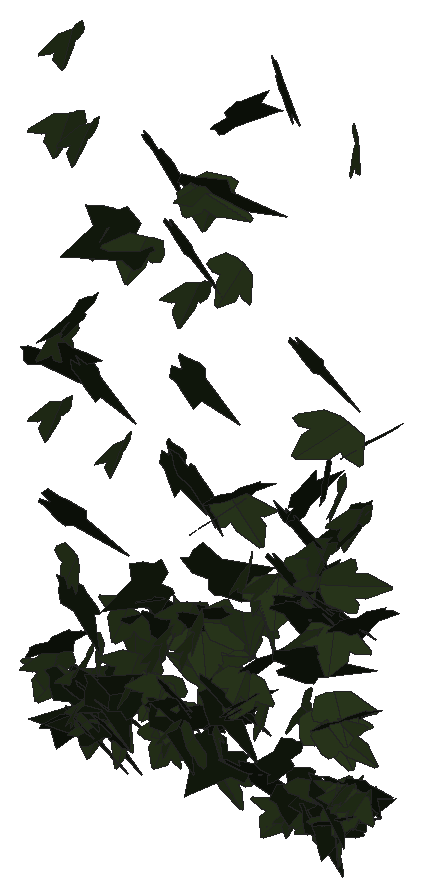
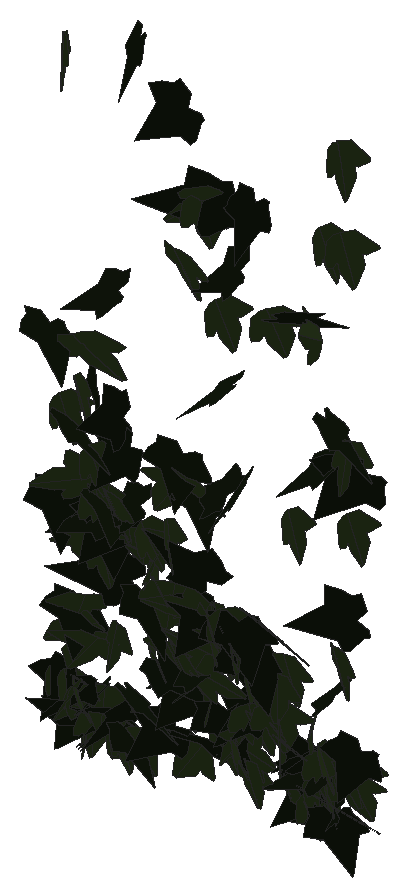
# SketchUp Ruby script. Lengths in inches.
U = 1.inch
M = Sketchup.active_model
def pt(a) = Geom::Point3d.new(a.map { |v| v * U })
def face(e, loops, mat)
  f = e.add_face(loops[0].map { |a| pt(a) })
  loops[1..].each { |l| e.add_face(l.map { |a| pt(a) }).erase! }
  f.material = f.back_material = mat if mat
  f
end
# faces: each face lists its corners as indices into pts; further lists are holes
def faces(e, pts, list, mat = nil) = list.each { |f| face(e, (f[0].is_a?(Array) ? f : [f]).map { |l| l.map { |i| pts[i] } }, mat) }
# xy, xz, yz: faces in a plane at the given z, y or x. An outline is a flat list of corners, or four numbers for a rectangle; further outlines are holes
def ring(l) = l.size == 4 ? [[l[0], l[1]], [l[2], l[1]], [l[2], l[3]], [l[0], l[3]]] : l.each_slice(2).to_a
def flat(e, list, mat, &to3) = list.each { |f| face(e, (f[0].is_a?(Array) ? f : [f]).map { |l| ring(l).map { |u, v| to3.(u, v) } }, mat) }
def xy(e, z, list, mat = nil) = flat(e, list, mat) { |x, y| [x, y, z] }
def xz(e, y, list, mat = nil) = flat(e, list, mat) { |x, z| [x, y, z] }
def yz(e, x, list, mat = nil) = flat(e, list, mat) { |y, z| [x, y, z] }
def lines(e, pts, list) = list.each { |a, b| e.add_line(pt(pts[a]), pt(pts[b])) }
# prism: a flat outline (further loops are holes) pulled along v
def prism(e, loops, v, mat = nil)
  f = face(e, loops, mat); d = Geom::Vector3d.new(v.map { |x| x * U })
  f.pushpull(f.normal.samedirection?(d) ? d.length : -d.length)
end
def box(e, o, s, mat = nil) = prism(e, [[o, [o[0] + s[0], o[1], o[2]], [o[0] + s[0], o[1] + s[1], o[2]], [o[0], o[1] + s[1], o[2]]]], [0, 0, s[2]], mat)
def at(x, y, z, deg = 0) = Geom::Transformation.translation(pt([x, y, z])) * Geom::Transformation.rotation(ORIGIN, Z_AXIS, deg.degrees)
def axes(o, x, y, z) = Geom::Transformation.new([*x, 0, *y, 0, *z, 0, *pt(o).to_a, 1])
def part(name) = M.definitions.add(name)
# library, detail: a bought-in or finely detailed component or shape, given as its bounding box
def library(name, o, s) = part(name).tap { |d| box(d.entities, o, s) }
def detail(e, o, s) = box(e.add_group.entities, o, s)
def put(e, d, t, mat = nil) = e.add_instance(d, t).tap { |i| i.material = mat if mat }
def group(e, t, mat = nil) = e.add_group.tap { |g| g.transformation = t; g.material = mat if mat }.entities
root = M.entities
M.materials.add("1026 AP 7946 SUNNY SIDE UP").color = [254, 231, 186]
M.materials.add("efeu1").color = [18, 25, 13]
M.materials.add("efeu2").color = [43, 57, 29]
c1 = part("ivyleaf_10")
p = [[0,0.5,-0.03],[-0.0625,2.02,-0.43],[-0.19,2.01,-0.46],[-0.54,1.05,-0.29],[-0.52,0.625,-0.18],[-0.83,0.76,-0.28],
  [-1.16,0.64,-0.33],[-1.15,0.33,-0.24],[-0.77,-0.39,0.02],[-0.3,-0.51,0.16],[0.04,-0.48,0.23],[-0.02,2.01,-0.4375],
  [-0.06,2.01,-0.43],[0.04,-0.49,0.23],[0.67,-0.49,0.14],[1.38,0.36,-0.2],[1.375,0.51,-0.24],[0.81,0.65,-0.19],
  [0.62,0.59,-0.15],[0.6,1.09,-0.28],[0.5,1.23,-0.31]]
faces(c1.entities,p,[[0,1,2,3,4,5,6,7,8,9,10],[11,12,0,13,14,15,16,17,18,19,20]],"efeu2")
c2 = part("ivyleaf_9")
p = [[1.54,2.16,1.25],[1.36,2.04,1.19],[-0.21,0.99,0.68],[-0.71,1.11,0.82],[-0.85,0.86,0.67],[-0.8,0.17,0.21],
  [-0.9,-0.01,0.1],[-0.67,-0.16,-0.02],[-0.08,-0.08,-0.05],[-0.03,-0.6,-0.4],[0.65,-0.88,-0.66],[0.83,-0.6,-0.49],
  [1.29,-0.42,-0.43],[1.8125,-0.07,-0.26],[1.21,0.44,0.15]]
faces(c2.entities,p,[[0,1,2,3,4,5,6,7,8,9,10,11,12,13,14]],"efeu1")
put(root,c1,axes([113.07,212.89,268.62],[-0.34334,-0.07653,0.12729],[-0.15139,-0.09188,-0.23364],[0.17197,-0.23369,0.04845]),"1026 AP 7946 SUNNY SIDE UP")
put(root,c2,axes([112.96,212.81,269.11],[0.15845,0.23705,0.05643],[0.06227,0.04104,-0.26432],[-0.37697,0.10642,-0.01995]),"1026 AP 7946 SUNNY SIDE UP")
put(root,c1,axes([113.02,212.83,268.85],[-0.17621,-0.24452,0.01132],[0.00626,-0.01543,-0.27699],[0.38492,-0.11169,0.00969]),"1026 AP 7946 SUNNY SIDE UP")
put(root,c1,axes([113.06,212.85,272.75],[-0.06958,-0.28014,0.02649],[-0.00163,-0.02748,-0.29232],[0.44258,-0.04414,0.00309]),"1026 AP 7946 SUNNY SIDE UP")
put(root,c2,axes([112.92,212.8125,273.57],[0.40205,0.1369,0.01777],[0.04671,-0.0208,-0.29705],[-0.21173,0.25537,-0.03179]),"1026 AP 7946 SUNNY SIDE UP")
put(root,c1,axes([113.18,212.87,277.2],[-0.16313,-0.28328,0.03071],[-0.00181,-0.03302,-0.3108],[0.44816,-0.10325,0.00992]),"1026 AP 7946 SUNNY SIDE UP")
put(root,c1,axes([113.14,212.82,273.87],[-0.08095,-0.26244,-0.12112],[0.06477,0.10995,-0.27427],[0.44654,-0.06352,0.01783]),"1026 AP 7946 SUNNY SIDE UP")
put(root,c2,axes([113.29,212.93,268.01],[0.07076,0.22691,-0.1179],[-0.02317,-0.11501,-0.23888],[-0.39986,0.04682,-0.00702]),"1026 AP 7946 SUNNY SIDE UP")
put(root,c2,axes([113.42,212.92,274.29],[-0.26406,0.22273,-0.07554],[0.04809,-0.07017,-0.28723],[-0.36619,-0.16983,0.01675]),"1026 AP 7946 SUNNY SIDE UP")
put(root,c1,axes([113.29,212.8,278.58],[-0.06665,-0.30699,-0.03908],[0.01318,0.03537,-0.31903],[0.48587,-0.04307,0.00329]),"1026 AP 7946 SUNNY SIDE UP")
put(root,c1,axes([113.35,212.78,270.5],[0.28252,-0.18935,-0.09053],[-0.04399,0.09166,-0.2651],[0.32456,0.17724,0.04287]),"1026 AP 7946 SUNNY SIDE UP")
put(root,c2,axes([113.02,212.85,271.23],[0.40541,-0.07099,0.12199],[0.16962,-0.05435,-0.27491],[0.13637,0.27864,-0.02074]),"1026 AP 7946 SUNNY SIDE UP")
put(root,c2,axes([113.21,212.91,268.62],[0.1171,-0.24383,-0.06473],[0.0273,0.06892,-0.25965],[0.39444,0.06762,0.03719]),"1026 AP 7946 SUNNY SIDE UP")
put(root,c1,axes([113.47,212.97,268.98],[0.08636,-0.25577,-0.01492],[-0.00783,0.01225,-0.26941],[0.40261,0.0551,-0.00204]),"1026 AP 7946 SUNNY SIDE UP")
put(root,c1,axes([113.47,212.83,268.35],[0.09709,-0.25754,-0.02951],[-0.00239,0.02758,-0.27262],[0.4072,0.06157,0.00543]),"1026 AP 7946 SUNNY SIDE UP")
put(root,c2,axes([113.79,212.85,268.17],[-0.33733,0.12121,0.10169],[-0.18391,-0.01491,-0.24479],[-0.16205,-0.23539,0.06612]),"1026 AP 7946 SUNNY SIDE UP")
put(root,c1,axes([113.52,212.875,277.17],[-0.02665,-0.30085,0.02682],[0.00126,-0.02783,-0.31058],[0.47506,-0.01681,0.00233]),"1026 AP 7946 SUNNY SIDE UP")
put(root,c2,axes([113.3125,212.93,269.96],[0.12745,-0.25297,0.03802],[0.00317,-0.03958,-0.2737],[0.40231,0.08045,-0.00989]),"1026 AP 7946 SUNNY SIDE UP")
put(root,c1,axes([113.58,212.88,268.8],[-0.18225,-0.23438,0.02402],[-0.00157,-0.02697,-0.26929],[0.37058,-0.11538,0.01067]),"1026 AP 7946 SUNNY SIDE UP")
put(root,c1,axes([113.67,212.87,268.39],[-0.07062,-0.25386,0.05692],[-0.01363,-0.05604,-0.26591],[0.40878,-0.04573,0.00097]),"1026 AP 7946 SUNNY SIDE UP")
put(root,c2,axes([113.39,212.87,268.07],[0.29729,-0.17873,0.03698],[0.05446,-0.01704,-0.26788],[0.28175,0.19188,0.01276]),"1026 AP 7946 SUNNY SIDE UP")
put(root,c1,axes([113.75,212.88,268.07],[-0.12803,-0.24599,0.03851],[-0.00362,-0.04005,-0.26696],[0.39156,-0.0808,0.01012]),"1026 AP 7946 SUNNY SIDE UP")
put(root,c1,axes([113.74,212.83,275.46],[0.17141,-0.14666,0.23722],[-0.14205,0.21554,0.18608],[-0.40627,-0.13724,0.03503]),"1026 AP 7946 SUNNY SIDE UP")
put(root,c2,axes([113.52,212.82,273.53],[0.33045,-0.17427,-0.09502],[-0.06233,0.09327,-0.27701],[0.30296,0.20927,0.04665]),"1026 AP 7946 SUNNY SIDE UP")
put(root,c2,axes([113.58,212.87,268.61],[0.35341,-0.14067,-0.01334],[0.04221,0.06499,-0.26329],[0.21797,0.2155,0.07261]),"1026 AP 7946 SUNNY SIDE UP")
put(root,c1,axes([113.7,212.96,269.18],[-0.02021,-0.03412,0.2681],[0.24776,-0.20962,-0.02151],[0.33044,0.15509,0.03253]),"1026 AP 7946 SUNNY SIDE UP")
put(root,c2,axes([114.2,213.01,275.72],[-0.35864,-0.09947,0.15449],[-0.17234,-0.11634,-0.25097],[0.22534,-0.24728,0.05393]),"1026 AP 7946 SUNNY SIDE UP")
put(root,c2,axes([113.78,212.79,268.54],[-0.13821,-0.02625,0.25803],[0.37194,-0.10009,0.07408],[0.13658,0.246,0.05937]),"1026 AP 7946 SUNNY SIDE UP")
put(root,c2,axes([113.84,212.8,268.17],[0.37975,-0.08446,-0.05098],[-0.08165,-0.00036,-0.26299],[0.13004,0.24643,-0.01625]),"1026 AP 7946 SUNNY SIDE UP")
put(root,c1,axes([114.07,212.92,272.48],[-0.01386,-0.27988,-0.02],[-0.00139,0.01786,-0.28837],[0.44097,-0.00874,-0.00154]),"1026 AP 7946 SUNNY SIDE UP")
put(root,c2,axes([113.9375,212.88,268.74],[0.0277,-0.25783,-0.06307],[-0.00826,0.05953,-0.26588],[0.41607,0.01835,-0.00108]),"1026 AP 7946 SUNNY SIDE UP")
put(root,c2,axes([114.35,212.86,268.85],[-0.39494,0.09218,0.00444],[-0.02265,-0.02831,-0.27387],[-0.14329,-0.2496,0.03103]),"1026 AP 7946 SUNNY SIDE UP")
put(root,c1,axes([114.32,212.79,270.04],[-0.39229,0.06098,0.10056],[-0.16882,-0.04153,-0.25711],[-0.06393,-0.26453,0.06188]),"1026 AP 7946 SUNNY SIDE UP")
put(root,c1,axes([114.16,212.85,268.17],[0.32041,-0.16362,0.04044],[0.06628,-0.01155,-0.2687],[0.2565,0.20737,0.01891]),"1026 AP 7946 SUNNY SIDE UP")
put(root,c1,axes([114.38,212.9,269.29],[-0.30986,-0.17049,0.05853],[-0.04637,-0.05395,-0.26788],[0.27923,-0.19815,0.02047]),"1026 AP 7946 SUNNY SIDE UP")
put(root,c1,axes([114.33,212.82,268.99],[0.06871,-0.22456,-0.144],[-0.00445,0.13998,-0.23392],[0.41484,0.0387,0.02134]),"1026 AP 7946 SUNNY SIDE UP")
put(root,c1,axes([114.38,213,275.64],[-0.2353,-0.23182,0.09243],[-0.00344,-0.10498,-0.27971],[0.39159,-0.14022,0.05308]),"1026 AP 7946 SUNNY SIDE UP")
put(root,c1,axes([114.44,212.86,269.74],[-0.40453,0.05586,0.05928],[-0.09489,-0.0091,-0.27038],[-0.08251,-0.2634,0.02031]),"1026 AP 7946 SUNNY SIDE UP")
put(root,c1,axes([114.81,212.88,268.5],[-0.06053,0.03023,-0.26723],[-0.25826,0.20127,0.05042],[0.3196,0.16837,-0.00987]),"1026 AP 7946 SUNNY SIDE UP")
put(root,c2,axes([114.8,212.85,270.63],[-0.39782,0.08932,-0.01565],[0.00665,-0.03486,-0.27471],[-0.14245,-0.25108,0.03089]),"1026 AP 7946 SUNNY SIDE UP")
put(root,c2,axes([114.83,212.87,270.06],[0.19796,0.17448,-0.16825],[-0.1412,-0.13774,-0.22237],[-0.3494,0.15452,-0.00547]),"1026 AP 7946 SUNNY SIDE UP")
put(root,c1,axes([114.74,212.89,269.03],[0.39604,-0.08266,-0.02171],[-0.04162,-0.01481,-0.27221],[0.12731,0.25228,-0.02145]),"1026 AP 7946 SUNNY SIDE UP")
put(root,c1,axes([114.82,212.87,269.68],[0.05128,-0.26694,0.02473],[0.0011,-0.02562,-0.27718],[0.42164,0.03253,-0.00228]),"1026 AP 7946 SUNNY SIDE UP")
put(root,c2,axes([114.79,212.88,277.28],[0.36497,-0.03585,-0.19508],[-0.29219,0.03576,-0.24168],[0.07916,0.29728,0.00734]),"1026 AP 7946 SUNNY SIDE UP")
put(root,c1,axes([114.84,212.875,269.11],[-0.2504,-0.20795,0.05208],[0.02163,-0.07425,-0.26425],[0.33625,-0.15008,0.05579]),"1026 AP 7946 SUNNY SIDE UP")
put(root,c1,axes([114.84,212.9,268.24],[0.36082,-0.10867,-0.0582],[-0.04474,0.06808,-0.25642],[0.18686,0.22615,0.05098]),"1026 AP 7946 SUNNY SIDE UP")
put(root,c2,axes([115.1,212.82,270.43],[0.19632,0.20326,-0.13399],[-0.15886,-0.09037,-0.24377],[-0.34566,0.15697,0.03593]),"1026 AP 7946 SUNNY SIDE UP")
put(root,c2,axes([114.88,212.8,269.14],[0.39048,-0.06735,-0.06722],[-0.10367,0.00444,-0.26473],[0.10426,0.25663,-0.01146]),"1026 AP 7946 SUNNY SIDE UP")
put(root,c1,axes([115.19,212.89,269.91],[0.21234,-0.08355,0.25324],[-0.30119,0.15577,0.16354],[-0.27662,-0.23373,0.01632]),"1026 AP 7946 SUNNY SIDE UP")
put(root,c1,axes([115.07,212.85,270.04],[0.03261,-0.27142,0.0217],[-0.00069,-0.0227,-0.28055],[0.42826,0.02063,-0.00211]),"1026 AP 7946 SUNNY SIDE UP")
put(root,c1,axes([115.1,212.83,268.5625],[0.04509,-0.26489,0.00432],[-0.00308,-0.00594,-0.27451],[0.4166,0.02862,-0.00249]),"1026 AP 7946 SUNNY SIDE UP")
put(root,c1,axes([115.02,212.79,268.7],[0.03963,0.22838,0.13842],[0.03114,0.13166,-0.23589],[-0.41445,0.03173,-0.00449]),"1026 AP 7946 SUNNY SIDE UP")
put(root,c2,axes([114.96,212.89,268.71],[0.08387,-0.25925,-0.01162],[0.00749,0.01099,-0.27251],[0.40786,0.05311,0.00739]),"1026 AP 7946 SUNNY SIDE UP")
put(root,c2,axes([115.03,212.83,272.67],[0.25397,-0.18707,-0.16613],[-0.17601,0.11489,-0.25381],[0.34496,0.19635,-0.00719]),"1026 AP 7946 SUNNY SIDE UP")
put(root,c2,axes([115.3125,212.8,268.92],[0.20368,0.14983,-0.18419],[-0.16757,-0.14501,-0.2046],[-0.32744,0.16741,-0.00987]),"1026 AP 7946 SUNNY SIDE UP")
put(root,c1,axes([115.33,212.85,270.43],[-0.16819,-0.24468,0.0482],[-0.00983,-0.04978,-0.27501],[0.392,-0.10623,0.01378]),"1026 AP 7946 SUNNY SIDE UP")
put(root,c1,axes([115.49,212.72,268.52],[-0.27498,0.12057,0.16103],[-0.25155,0.03428,-0.21235],[-0.1804,-0.23158,0.05065]),"1026 AP 7946 SUNNY SIDE UP")
put(root,c2,axes([115.06,212.9,276.13],[0.32608,-0.21219,0.001],[-0.01353,-0.01144,-0.30538],[0.3334,0.20707,-0.01337]),"1026 AP 7946 SUNNY SIDE UP")
put(root,c1,axes([115.39,212.87,275.36],[-0.11027,-0.27928,0.06563],[-0.00027,-0.06717,-0.29659],[0.45097,-0.06832,0.01587]),"1026 AP 7946 SUNNY SIDE UP")
put(root,c1,axes([115.43,212.85,270.05],[0.04035,-0.26985,0.03235],[-0.0041,-0.03332,-0.27938],[0.42744,0.02515,-0.00573]),"1026 AP 7946 SUNNY SIDE UP")
put(root,c1,axes([115.74,212.88,269.47],[0.01117,-0.03601,-0.31079],[-0.4185,0.14439,-0.02338],[0.22976,0.26475,-0.02748]),"1026 AP 7946 SUNNY SIDE UP")
put(root,c2,axes([115.25,212.95,272.5],[0.1723,-0.26197,0.10891],[0.06079,-0.10003,-0.29311],[0.44091,0.11617,-0.00215]),"1026 AP 7946 SUNNY SIDE UP")
put(root,c2,axes([115.33,212.76,274.13],[0.29185,-0.17538,-0.13269],[-0.06142,0.13843,-0.25333],[0.33565,0.17783,0.06902]),"1026 AP 7946 SUNNY SIDE UP")
put(root,c1,axes([115.53,212.88,270.39],[0.12398,-0.24599,0.08679],[0.07105,-0.07521,-0.26583],[0.40336,0.08886,0.02014]),"1026 AP 7946 SUNNY SIDE UP")
put(root,c1,axes([115.48,212.9,270.0625],[0.42062,0.11601,0.04379],[0.0762,-0.00696,-0.29927],[-0.17832,0.27066,-0.02459]),"1026 AP 7946 SUNNY SIDE UP")
put(root,c1,axes([115.71,212.875,276.95],[-0.20849,-0.2677,0.03289],[0.00112,-0.03762,-0.30746],[0.4242,-0.13147,0.01698]),"1026 AP 7946 SUNNY SIDE UP")
put(root,c2,axes([115.59,212.79,270.45],[0.34602,0.16328,0.0102],[0.03692,-0.01665,-0.28098],[-0.25446,0.21961,-0.02689]),"1026 AP 7946 SUNNY SIDE UP")
put(root,c1,axes([115.74,212.78,268.94],[-0.24455,0.21087,-0.02553],[0.008,-0.0285,-0.26978],[-0.33398,-0.15509,0.01224]),"1026 AP 7946 SUNNY SIDE UP")
put(root,c2,axes([115.87,212.9375,268.39],[-0.38103,-0.09607,-0.02487],[0.06059,-0.03417,-0.26457],[0.14327,-0.24106,0.04575]),"1026 AP 7946 SUNNY SIDE UP")
put(root,c1,axes([115.6,212.77,277.02],[-0.20729,-0.15161,-0.23889],[0.34871,0.09466,-0.19381],[0.25922,-0.24858,0.06969]),"1026 AP 7946 SUNNY SIDE UP")
put(root,c2,axes([115.97,212.66,272.17],[-0.01216,0.2722,0.04176],[-0.01039,0.03881,-0.28024],[-0.43225,-0.00859,0.00556]),"1026 AP 7946 SUNNY SIDE UP")
put(root,c1,axes([115.53,212.9,269.8],[0.13728,-0.03787,-0.25994],[0.39922,-0.01111,0.09224],[-0.03614,-0.26656,0.0315]),"1026 AP 7946 SUNNY SIDE UP")
put(root,c2,axes([115.49,212.78,276.96],[0.34205,0.00281,0.22152],[0.33779,0.01039,-0.22399],[-0.01463,0.30568,0.00736]),"1026 AP 7946 SUNNY SIDE UP")
put(root,c1,axes([115.84,212.88,268.15],[-0.37565,0.05719,-0.0943],[0.12982,-0.04757,-0.252],[-0.10998,-0.25149,0.02463]),"1026 AP 7946 SUNNY SIDE UP")
put(root,c2,axes([115.66,212.91,271.01],[-0.02772,0.01337,0.27992],[0.38837,-0.11317,0.02159],[0.17903,0.24757,-0.0035]),"1026 AP 7946 SUNNY SIDE UP")
put(root,c2,axes([115.76,212.8125,269.48],[0.32806,-0.17179,-0.03563],[0.01866,0.06605,-0.27152],[0.27461,0.20074,0.06101]),"1026 AP 7946 SUNNY SIDE UP")
put(root,c2,axes([115.85,212.84,269.21],[0.17041,-0.2417,-0.05275],[0.00133,0.05479,-0.27155],[0.38804,0.10595,0.0241]),"1026 AP 7946 SUNNY SIDE UP")
put(root,c2,axes([116.04,212.76,269.01],[0.18052,0.2043,0.12993],[0.09206,0.11043,-0.24076],[-0.36514,0.12884,0.00353]),"1026 AP 7946 SUNNY SIDE UP")
put(root,c1,axes([115.82,212.86,270.37],[-0.07395,-0.00397,0.27825],[0.32083,0.17917,0.04036],[-0.2784,0.20754,-0.0274]),"1026 AP 7946 SUNNY SIDE UP")
put(root,c1,axes([116.15,212.82,275.93],[0.39463,-0.15499,-0.05184],[-0.07053,0.02145,-0.3037],[0.2459,0.25489,-0.00391]),"1026 AP 7946 SUNNY SIDE UP")
put(root,c1,axes([116.14,212.89,269.66],[0.32411,-0.17106,0.02156],[0.00612,-0.0295,-0.27534],[0.2711,0.20517,-0.01956]),"1026 AP 7946 SUNNY SIDE UP")
put(root,c2,axes([116.25,212.65,272.64],[0.14125,0.26165,0.02823],[-0.01062,0.02968,-0.28434],[-0.41329,0.08866,0.01696]),"1026 AP 7946 SUNNY SIDE UP")
put(root,c2,axes([116.09,212.78,278.32],[0.18052,0.19867,0.21105],[0.20084,0.16034,-0.23428],[-0.39984,0.17023,-0.0224]),"1026 AP 7946 SUNNY SIDE UP")
put(root,c1,axes([116.23,212.91,270.57],[-0.41983,-0.05824,-0.01248],[0.02649,-0.02218,-0.28045],[0.08959,-0.26634,0.02444]),"1026 AP 7946 SUNNY SIDE UP")
put(root,c2,axes([116.4,212.9375,269.41],[-0.18306,0.16666,-0.17632],[0.02676,-0.1851,-0.19761],[-0.37574,-0.09438,0.07183]),"1026 AP 7946 SUNNY SIDE UP")
put(root,c1,axes([116.37,212.77,271.46],[0.05298,-0.2602,-0.0989],[-0.00969,0.09449,-0.26968],[0.4352,0.03378,0.00603]),"1026 AP 7946 SUNNY SIDE UP")
put(root,c1,axes([116.29,212.85,269.66],[0.41791,-0.02043,-0.01428],[-0.02475,-0.02632,-0.27331],[0.02977,0.26483,-0.02669]),"1026 AP 7946 SUNNY SIDE UP")
put(root,c1,axes([116.14,212.8125,272.32],[0.3406,0.10758,0.14316],[0.16322,0.09847,-0.24573],[-0.22203,0.23741,0.03896]),"1026 AP 7946 SUNNY SIDE UP")
put(root,c2,axes([116.3,212.8,268.35],[0.4136,0.02078,-0.00489],[-0.00736,-0.00254,-0.27183],[-0.03274,0.26307,-0.00069]),"1026 AP 7946 SUNNY SIDE UP")
put(root,c1,axes([116.55,212.875,270.67],[0.23052,-0.22298,0.06564],[0.05257,-0.05578,-0.27522],[0.36139,0.15035,-0.00183]),"1026 AP 7946 SUNNY SIDE UP")
put(root,c1,axes([116.59,212.86,269.39],[0.23818,-0.22269,0.00194],[0.02399,0.00658,-0.2769],[0.34936,0.15136,0.01769]),"1026 AP 7946 SUNNY SIDE UP")
put(root,c2,axes([116.77,212.79,270.25],[-0.01086,0.26992,-0.04639],[-0.00425,-0.04664,-0.27841],[-0.43067,-0.00635,0.00392]),"1026 AP 7946 SUNNY SIDE UP")
put(root,c1,axes([116.71,212.86,271.35],[-0.03217,-0.27079,0.05998],[-0.01523,-0.05919,-0.28006],[0.43577,-0.02206,-0.00536]),"1026 AP 7946 SUNNY SIDE UP")
put(root,c1,axes([116.67,212.8,270.86],[-0.16574,0.25726,0.01194],[-0.02889,0.0034,-0.28593],[-0.40379,-0.10584,0.01556]),"1026 AP 7946 SUNNY SIDE UP")
put(root,c2,axes([117,212.88,268.69],[-0.27714,0.19531,0.00347],[-0.04682,-0.02386,-0.26831],[-0.30354,-0.17464,0.03822]),"1026 AP 7946 SUNNY SIDE UP")
put(root,c1,axes([117.06,212.84,267.92],[-0.30907,-0.10543,0.1447],[-0.1721,-0.09246,-0.22886],[0.21693,-0.22357,0.02459]),"1026 AP 7946 SUNNY SIDE UP")
put(root,c2,axes([116.88,212.83,279.16],[0.28617,-0.12302,-0.22751],[-0.31033,0.09953,-0.2248],[0.24686,0.26773,-0.01886]),"1026 AP 7946 SUNNY SIDE UP")
put(root,c1,axes([116.82,212.85,271.28],[0.38905,0.12878,-0.00446],[0.00839,-0.02119,-0.28664],[-0.20247,0.24657,-0.02046]),"1026 AP 7946 SUNNY SIDE UP")
put(root,c2,axes([117.11,212.84,268.04],[-0.13041,0.2392,-0.05689],[0.02271,-0.05487,-0.26109],[-0.38582,-0.08408,0.00386]),"1026 AP 7946 SUNNY SIDE UP")
put(root,c1,axes([117.14,212.91,267.98],[-0.03131,-0.25925,0.00166],[-0.0124,-0.00249,-0.26776],[0.40749,-0.01999,-0.00802]),"1026 AP 7946 SUNNY SIDE UP")
put(root,c2,axes([116.91,212.82,271.68],[0.32211,-0.19315,0.01196],[0.03788,0.00709,-0.28915],[0.302,0.20512,0.02351]),"1026 AP 7946 SUNNY SIDE UP")
put(root,c1,axes([117.22,212.89,269.57],[-0.02171,-0.19374,-0.19351],[0.02036,0.18629,-0.19901],[0.42262,-0.01893,-0.00035]),"1026 AP 7946 SUNNY SIDE UP")
put(root,c2,axes([117.1,212.8,268.36],[0.13845,-0.1007,-0.25391],[-0.12414,0.23743,-0.1279],[0.39894,0.10883,0.04832]),"1026 AP 7946 SUNNY SIDE UP")
put(root,c1,axes([117.29,212.9,271.66],[0.31888,-0.17503,-0.07411],[-0.07827,0.05088,-0.27561],[0.28647,0.20874,0.00719]),"1026 AP 7946 SUNNY SIDE UP")
put(root,c2,axes([117.41,212.87,271.48],[0.04061,0.2054,0.19373],[-0.06922,0.18835,-0.20588],[-0.43113,-0.01089,0.0513]),"1026 AP 7946 SUNNY SIDE UP")
put(root,c2,axes([117.13,212.77,272.51],[0.43473,-0.09145,-0.08387],[-0.13486,-0.00296,-0.29856],[0.13663,0.28805,-0.02784]),"1026 AP 7946 SUNNY SIDE UP")
put(root,c2,axes([117.29,212.74,271.33],[0.35261,0.16906,0.0205],[0.04086,-0.00308,-0.28873],[-0.26435,0.22502,-0.01729]),"1026 AP 7946 SUNNY SIDE UP")
put(root,c2,axes([117.48,212.7,271.24],[0.26122,0.17864,-0.12832],[-0.15705,-0.07815,-0.25111],[-0.30533,0.19303,0.01938]),"1026 AP 7946 SUNNY SIDE UP")
put(root,c2,axes([117.36,212.625,272.85],[0.0667,0.10653,0.29168],[0.23485,0.24055,-0.11514],[-0.41262,0.15413,-0.01838]),"1026 AP 7946 SUNNY SIDE UP")
put(root,c1,axes([117.51,212.84,268.46],[-0.34975,-0.13589,-0.01335],[0.02965,-0.00753,-0.26804],[0.21247,-0.22263,0.01542]),"1026 AP 7946 SUNNY SIDE UP")
put(root,c1,axes([117.53,212.82,270.8125],[-0.10683,-0.26932,0.007],[0.01093,-0.01033,-0.28604],[0.42354,-0.06767,0.00915]),"1026 AP 7946 SUNNY SIDE UP")
put(root,c2,axes([117.22,212.93,275.06],[0.33047,-0.20181,-0.004],[0.03025,0.02397,-0.29837],[0.3159,0.20882,0.03276]),"1026 AP 7946 SUNNY SIDE UP")
put(root,c1,axes([117.57,212.87,271.6],[-0.19746,-0.24488,0.04542],[0.0143,-0.0554,-0.28179],[0.39137,-0.12152,0.03321]),"1026 AP 7946 SUNNY SIDE UP")
put(root,c2,axes([117.23,212.66,270.32],[0.23861,0.02097,0.25269],[0.37626,0.05451,-0.15707],[-0.09012,0.28313,0.01325]),"1026 AP 7946 SUNNY SIDE UP")
put(root,c1,axes([117.66,212.86,272.24],[-0.09198,-0.27413,0.03305],[0.00247,-0.03471,-0.28883],[0.43427,-0.05786,0.00865]),"1026 AP 7946 SUNNY SIDE UP")
put(root,c2,axes([117.48,212.93,267.98],[0.13057,-0.24196,-0.0201],[-0.02701,0.01326,-0.26317],[0.38057,0.08395,-0.01178]),"1026 AP 7946 SUNNY SIDE UP")
put(root,c2,axes([117.37,212.875,271.41],[0.38189,-0.13533,-0.00692],[0.05098,0.06993,-0.27485],[0.2068,0.23266,0.08053]),"1026 AP 7946 SUNNY SIDE UP")
put(root,c1,axes([117.67,212.84,268],[-0.17315,-0.22707,-0.03658],[0.05039,0.02238,-0.25912],[0.35754,-0.11312,0.01881]),"1026 AP 7946 SUNNY SIDE UP")
put(root,c1,axes([117.81,212.91,274.04],[0.40888,0.03347,-0.18257],[-0.27362,-0.0364,-0.27005],[-0.07562,0.31268,-0.01002]),"1026 AP 7946 SUNNY SIDE UP")
put(root,c2,axes([117.81,212.64,273.22],[0.02891,-0.00893,0.29217],[0.06441,0.28136,0.00804],[-0.44157,0.04046,0.0203]),"1026 AP 7946 SUNNY SIDE UP")
put(root,c1,axes([117.53,213.05,269.39],[0.34424,0.17663,0.12386],[0.17744,0.0489,-0.28783],[-0.28424,0.24444,-0.02968]),"1026 AP 7946 SUNNY SIDE UP")
put(root,c2,axes([117.72,212.99,268.2],[-0.24225,-0.2026,-0.03641],[0.06959,0.00901,-0.26039],[0.31549,-0.15756,0.02948]),"1026 AP 7946 SUNNY SIDE UP")
put(root,c2,axes([117.64,212.95,268.39],[0.07414,-0.24482,0.07372],[0.01399,-0.07257,-0.25723],[0.40144,0.04774,-0.00465]),"1026 AP 7946 SUNNY SIDE UP")
put(root,c1,axes([117.87,212.95,268.39],[-0.07913,-0.22912,0.11236],[-0.00994,-0.11135,-0.24176],[0.39977,-0.04812,0.01623]),"1026 AP 7946 SUNNY SIDE UP")
put(root,c1,axes([117.77,212.88,270.89],[0.36134,0.14548,-0.02366],[-0.01355,-0.03073,-0.27951],[-0.23139,0.22898,-0.02058]),"1026 AP 7946 SUNNY SIDE UP")
put(root,c1,axes([117.88,212.93,268.51],[0.10694,-0.25128,0.02733],[0.00547,-0.02801,-0.26831],[0.39751,0.06798,-0.00366]),"1026 AP 7946 SUNNY SIDE UP")
put(root,c1,axes([117.78,212.97,267.8],[-0.10284,0.08263,-0.23831],[0.09277,-0.22758,-0.10206],[-0.37565,-0.07883,0.04003]),"1026 AP 7946 SUNNY SIDE UP")
put(root,c1,axes([117.97,212.79,273.2],[0.12393,-0.26989,-0.07135],[-0.03071,0.06485,-0.28927],[0.43645,0.0812,-0.0001]),"1026 AP 7946 SUNNY SIDE UP")
put(root,c2,axes([117.99,212.77,269.69],[0.13723,0.25404,0.03725],[-0.02384,0.04172,-0.27501],[-0.40246,0.08415,0.02899]),"1026 AP 7946 SUNNY SIDE UP")
put(root,c2,axes([118.14,212.92,272.73],[-0.28393,0.21106,-0.04443],[0.01804,-0.04832,-0.2855],[-0.33863,-0.17954,0.02204]),"1026 AP 7946 SUNNY SIDE UP")
put(root,c2,axes([117.89,212.76,268.1],[0.25677,0.18878,0.05747],[0.01493,0.06347,-0.25444],[-0.30869,0.1601,0.0355]),"1026 AP 7946 SUNNY SIDE UP")
put(root,c1,axes([117.88,212.9,268.42],[0.01107,-0.15172,-0.2201],[0.1334,0.20267,-0.14479],[0.38868,-0.06523,0.05596]),"1026 AP 7946 SUNNY SIDE UP")
put(root,c1,axes([117.86,212.86,269.87],[0.26894,0.20846,0.02925],[0.05104,0.00846,-0.277],[-0.3266,0.17298,-0.01921]),"1026 AP 7946 SUNNY SIDE UP")
put(root,c2,axes([117.75,212.89,267.99],[0.00508,0.02548,0.268],[0.38854,0.08409,-0.01116],[-0.13331,0.24605,-0.02231]),"1026 AP 7946 SUNNY SIDE UP")
put(root,c1,axes([118.04,212.97,268.58],[-0.01358,-0.2594,-0.01802],[0.0034,0.01596,-0.26728],[0.40864,-0.00875,0.00162]),"1026 AP 7946 SUNNY SIDE UP")
put(root,c2,axes([117.96,212.92,268.64],[0.36442,0.108,-0.02858],[-0.03535,-0.01886,-0.2634],[-0.17197,0.23273,-0.00642]),"1026 AP 7946 SUNNY SIDE UP")
put(root,c1,axes([117.84,212.79,269.44],[0.2302,0.06949,0.22397],[0.27887,0.12721,-0.16448],[-0.22497,0.22879,0.0253]),"1026 AP 7946 SUNNY SIDE UP")
put(root,c1,axes([118.1,212.85,268.49],[0.42231,-0.08894,-0.01435],[-0.03156,-0.01805,-0.29057],[0.13787,0.26831,-0.02256]),"1026 AP 7946 SUNNY SIDE UP")
put(root,c1,axes([117.94,212.74,271.75],[0.00611,0.01987,0.31646],[0.16606,0.28836,-0.01891],[-0.45446,0.10563,-0.00266]),"1026 AP 7946 SUNNY SIDE UP")
put(root,c1,axes([118.2,212.86,272.88],[-0.08404,-0.27778,0.04382],[0.00622,-0.04564,-0.2914],[0.44221,-0.05215,0.01243]),"1026 AP 7946 SUNNY SIDE UP")
put(root,c1,axes([118.2,212.82,278.62],[0.18207,-0.25994,-0.11205],[0.05032,0.12746,-0.28179],[0.4393,0.09313,0.07872]),"1026 AP 7946 SUNNY SIDE UP")
put(root,c1,axes([118.28,212.89,268.55],[-0.05933,-0.26014,0.01592],[0.00772,-0.01781,-0.2708],[0.40984,-0.03732,0.00741]),"1026 AP 7946 SUNNY SIDE UP")
put(root,c2,axes([118.31,212.76,271.375],[0.11891,0.26397,-0.01739],[-0.00118,-0.0189,-0.28295],[-0.41607,0.0755,-0.00416]),"1026 AP 7946 SUNNY SIDE UP")
put(root,c2,axes([118.42,212.9,274.08],[0.00264,0.28204,0.04695],[-0.0392,0.04395,-0.28917],[-0.44713,-0.00219,0.02563]),"1026 AP 7946 SUNNY SIDE UP")
